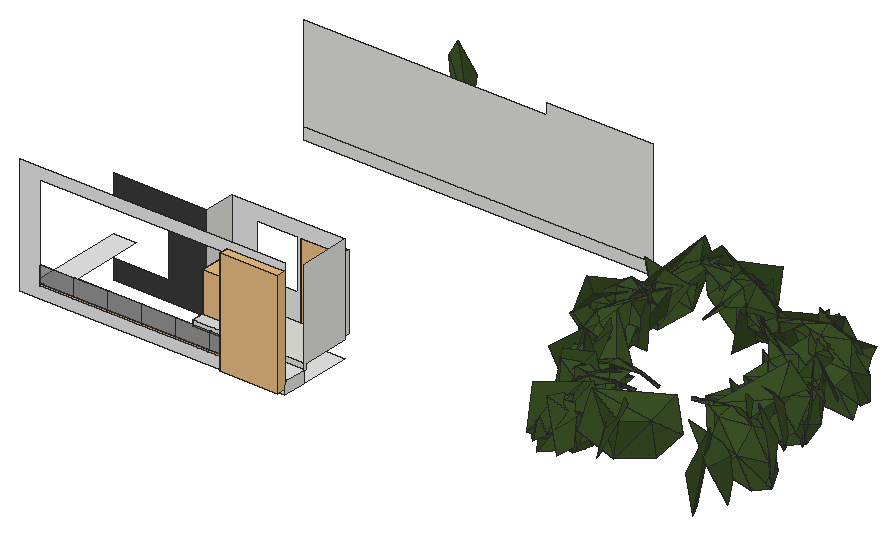
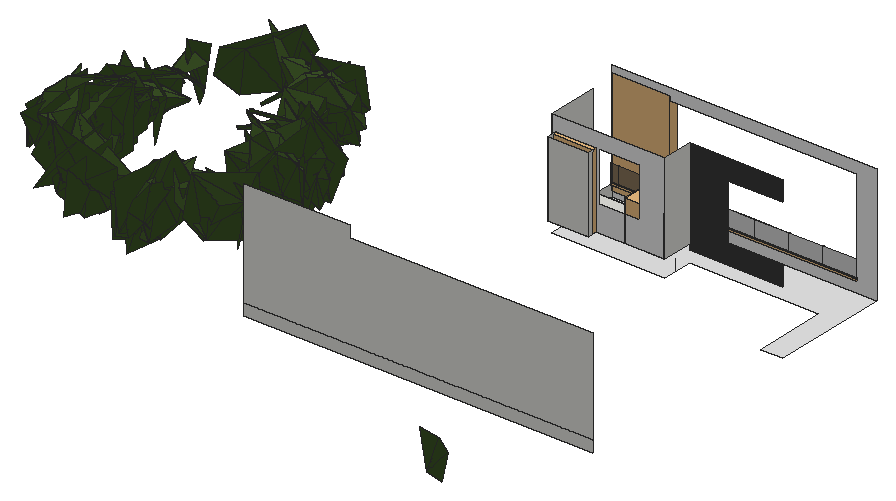
# SketchUp Ruby script. Lengths in inches.
U = 1.inch
M = Sketchup.active_model
def pt(a) = Geom::Point3d.new(a.map { |v| v * U })
def face(e, loops, mat)
  f = e.add_face(loops[0].map { |a| pt(a) })
  loops[1..].each { |l| e.add_face(l.map { |a| pt(a) }).erase! }
  f.material = f.back_material = mat if mat
  f
end
# faces: each face lists its corners as indices into pts; further lists are holes
def faces(e, pts, list, mat = nil) = list.each { |f| face(e, (f[0].is_a?(Array) ? f : [f]).map { |l| l.map { |i| pts[i] } }, mat) }
# xy, xz, yz: faces in a plane at the given z, y or x. An outline is a flat list of corners, or four numbers for a rectangle; further outlines are holes
def ring(l) = l.size == 4 ? [[l[0], l[1]], [l[2], l[1]], [l[2], l[3]], [l[0], l[3]]] : l.each_slice(2).to_a
def flat(e, list, mat, &to3) = list.each { |f| face(e, (f[0].is_a?(Array) ? f : [f]).map { |l| ring(l).map { |u, v| to3.(u, v) } }, mat) }
def xy(e, z, list, mat = nil) = flat(e, list, mat) { |x, y| [x, y, z] }
def xz(e, y, list, mat = nil) = flat(e, list, mat) { |x, z| [x, y, z] }
def yz(e, x, list, mat = nil) = flat(e, list, mat) { |y, z| [x, y, z] }
def lines(e, pts, list) = list.each { |a, b| e.add_line(pt(pts[a]), pt(pts[b])) }
# prism: a flat outline (further loops are holes) pulled along v
def prism(e, loops, v, mat = nil)
  f = face(e, loops, mat); d = Geom::Vector3d.new(v.map { |x| x * U })
  f.pushpull(f.normal.samedirection?(d) ? d.length : -d.length)
end
def box(e, o, s, mat = nil) = prism(e, [[o, [o[0] + s[0], o[1], o[2]], [o[0] + s[0], o[1] + s[1], o[2]], [o[0], o[1] + s[1], o[2]]]], [0, 0, s[2]], mat)
def at(x, y, z, deg = 0) = Geom::Transformation.translation(pt([x, y, z])) * Geom::Transformation.rotation(ORIGIN, Z_AXIS, deg.degrees)
def axes(o, x, y, z) = Geom::Transformation.new([*x, 0, *y, 0, *z, 0, *pt(o).to_a, 1])
def part(name) = M.definitions.add(name)
# library, detail: a bought-in or finely detailed component or shape, given as its bounding box
def library(name, o, s) = part(name).tap { |d| box(d.entities, o, s) }
def detail(e, o, s) = box(e.add_group.entities, o, s)
def put(e, d, t, mat = nil) = e.add_instance(d, t).tap { |i| i.material = mat if mat }
def group(e, t, mat = nil) = e.add_group.tap { |g| g.transformation = t; g.material = mat if mat }.entities
root = M.entities
M.materials.add("AM113_062_Tilia").color = [58, 81, 37]
M.materials.add("[Color M07]").color = [58, 58, 58]
M.materials.add("[Translucent_Glass_Blue]").color = [63, 63, 63]
M.materials["[Translucent_Glass_Blue]"].alpha = 0.35
M.materials.add("metal railing").color = [165, 165, 165]
M.materials.add("plastic2").color = [86, 86, 86]
M.materials.add("white_wall").color = [233, 233, 233]
c1 = library("Railing",[0,0,0],[72,2.52,4.03])
c2 = part("railing plastic")
box(c2.entities,[0,0.75,0],[72,0.26,0.68],"plastic2")
box(c2.entities,[0,0,0],[72,0.26,0.68],"plastic2")
c3 = part("Glass Railing pro")
put(c3.entities,c1,axes([0,0,0],[7.25965,0,0],[0,1,0],[0,0,1]))
put(c3.entities,c2,axes([0,0.75,3.47],[7.25965,0,0],[0,1,0],[0,0,1]))
c4 = part("sheet glass")
box(c4.entities,[0,0,0],[39.37,0.39,39.37],"[Translucent_Glass_Blue]")
c5 = part("glass stretch")
box(c5.entities,[0,0,0],[39.37,0.39,43.31],"[Translucent_Glass_Blue]")
c6 = part("glass frame")
put(c6.entities,c4,axes([0,0,0],[1.8288,0,0],[0,1.016,0],[0,0,1]))
put(c6.entities,c5,axes([505.4,0,0],[0.43929,0,0],[0,1.016,0],[0,0,0.90909]))
put(c6.entities,c4,axes([72.2,0,0],[1.8288,0,0],[0,1.016,0],[0,0,1]))
put(c6.entities,c4,axes([144.4,0,0],[1.8288,0,0],[0,1.016,0],[0,0,1]))
put(c6.entities,c4,axes([216.6,0,0],[1.8288,0,0],[0,1.016,0],[0,0,1]))
put(c6.entities,c4,axes([288.8,0,0],[1.8288,0,0],[0,1.016,0],[0,0,1]))
put(c6.entities,c4,axes([361,0,0],[1.8288,0,0],[0,1.016,0],[0,0,1]))
put(c6.entities,c4,axes([433.2,0,0],[1.8288,0,0],[0,1.016,0],[0,0,1]))
c7 = part("Glass Railing +")
put(c7.entities,c3,at(0,0,0),"metal railing")
put(c7.entities,c6,at(0,1.0625,1.53),"metal railing")
c8 = part("My+Glass_Railing")
put(c8.entities,c7,at(-0.34,0,0))
c9 = library("plant (1)",[-21.34,-27.21,-0.38],[41.91,41.15,38.97])
c10 = library("Shrub+_Grass",[-121.83,-22.34,0],[123.96,19.94,123.95])
c11 = library("PINTU+6+YA",[0,-0.6875,0],[35.83,8.07,80.71])
xy(root,273.04,[[371.87,28.625,371.87,278.26,418.81,278.26,418.81,121.6875,695.48,121.6875,695.48,187.1875,935.92,187.1875,935.92,28.625]],"white_wall")
xy(root,308.91,[[695.48,83.29,935.92,83.29,935.92,187.1875,927.68,187.1875,927.68,207.4375,841.77,207.4375,841.77,187.1875,695.48,187.1875]])
xz(root,28.625,[[371.87,273.04,935.92,273.04,935.92,297.35,413.32,297.35,413.32,500.91,935.92,500.91,935.92,525.1,371.87,525.1]],"white_wall")
xz(root,83.29,[[695.48,297.35,935.92,308.91]])
xz(root,121.6875,[[496.21,297.35,695.48,297.35,695.48,500.91,496.21,500.91,496.21,457.89,613.65,457.89,613.65,339.36,496.21,339.36]],"[Color M07]")
xz(root,187.1875,[[695.48,308.91,841.77,308.91,841.77,469.24,835.24,469.24,835.24,364.43,748.74,364.43,748.74,469.24,927.68,469.24,927.68,308.91,935.92,308.91,935.92,500.91,695.48,500.91]],"white_wall")
xz(root,207.4375,[[841.77,308.91,927.68,469.24]])
xz(root,725.65,[[418.81,273.04,1160.625,297.35],[418.81,297.35,418.81,500.91,935.92,500.91,935.92,525.1,1160.625,525.1,1160.625,297.35]])
yz(root,695.48,[[83.29,297.35,121.6875,308.91],[121.6875,308.91,187.1875,500.91]])
yz(root,841.77,[[187.1875,308.91,207.4375,469.24]])
yz(root,927.68,[[187.1875,308.91,207.4375,469.24]])
yz(root,935.92,[[28.625,273.04,76.875,297.35],[76.875,297.35,76.875,500.91,187.1875,500.91,187.1875,308.91,83.29,308.91,83.29,297.35]])
p = [[1726.04,425.28,347.14],[1633.73,427.27,429.39],[1677.65,428,251.14],[1612.37,455.72,310.63],[1284.72,331.65,346.32],[1334.89,406.05,429.43],
  [1303.44,377.73,253.56],[1361.71,418.12,309.96],[1703.03,155.11,256.72],[1686.97,186.29,255.56],[1681.79,228.74,364.75],[1365.41,276.39,256.16],
  [1387.28,221.24,314.07],[1379.55,269.8,365.5],[1360.82,315.08,327.84],[1397.36,380.08,315.61],[1345.32,356.24,258.76],[1690.04,216.5,392.49],
  [1699.77,139.08,344.57],[1721.375,172.58,346.28],[1726.25,219.67,257.36],[1704.02,272.17,325.3],[1717.7,253.93,333.4375],[1741.12,263.69,269.3],
  [1749.15,306.62,257.48],[1745.96,302.05,307.52],[1737.48,337.56,274.56],[1758.18,295.16,270.1],[1723.52,296.66,263.39],[1676.53,340.13,353.67],
  [597.55,943.93,270.1],[562.89,945.4375,263.39],[515.91,988.9,353.67],[1428.98,246.7,383.67],[1431.46,209.37,265.86],[1381.28,141.36,270.84],
  [1342.81,341.56,313.11],[1318.22,305.65,268.03],[1318.72,262.98,284.91],[1357.34,354.46,274.22],[1301.16,337.16,269.15],[1322.875,316.55,292.7],
  [1288.6,336.99,316.2],[1276.45,388.35,348.44],[1280.3,374.92,279.89],[1696.57,232,309],[1600.74,380.24,382.82],[1642.35,361.07,270.04],
  [1696.99,298.53,290.85],[1689.04,347.97,381.4],[1763.05,306.88,358.94],[528.41,996.75,381.4],[602.42,955.65,358.94],[1679.3,390.71,342.86],
  [1690.81,406.47,275.41],[1714.71,443.96,270.55],[1719.99,428.79,316.66],[1722.2,471.07,298.74],[1393.48,140.27,384.3125],[1301.2,301.36,352.37],
  [1350.83,325.49,273.55],[1396.78,333.4,351.65],[1470.81,570.52,383.75],[1429.89,600.59,274.58],[1442.08,684.31,273.91],[1451.84,681.07,387.71],
  [1407.09,344.35,313.43],[1716.59,344.22,341.74],[1679.02,375.96,340.52],[1450.08,141.61,377.59],[1398.19,150.79,345.67],[1433.36,171.22,274.86],
  [1493.32,149.93,318.77],[1356.96,199,367.41],[1352.15,178.13,289],[1707.07,471.59,421.7],[1747.09,414.05,356.48],[1719.76,427.52,275.13],
  [1687.28,476.17,400.61],[1689.53,443.21,285.93],[1646.43,385.33,325.7],[1338.36,322.47,413.4],[1265.81,318.08,356.36],[1284.91,340.12,275.76],
  [1350.19,338.7,392.76],[1313.27,358.45,285.1],[1579.47,670.33,379.39],[1600.1875,656.35,276.45],[1549.98,598.59,293.16],[1631.46,604.85,285.62],
  [1559.9,610.85,276.43],[1568.6875,638.62,349.05],[1514.9,622.74,311.54],[1640.95,624.18,294.44],[1568.94,637.52,277.53],[1570.34,627.16,358.07],
  [1522.17,639.52,309.81],[1676.7,375.7,357.375],[1660.27,387.38,278.41],[1646.98,467.65,293.93],[1308.26,276.26,291.07],[1341.96,277.58,278.61],
  [1402.26,280.86,372.95],[1507.2,646.41,353.86],[1487.34,665.98,278.91],[1412.2,633.41,288.58],[1416.23,156.82,278.97],[1477.17,126.84,318.15],
  [1448.93,154.68,381.79],[1399.95,178.18,359.37],[1383.45,251.52,359.07],[1350.8125,202.68,304.82],[1335.69,376,279.71],[1375.93,318.09,305.31],
  [1338.23,326.37,368.4375],[1303.43,369.125,354.66],[1300.6875,433.48,401.69],[1277.03,424.43,315.95],[1286.06,420.29,333.45],[1626.25,386.16,394.92],
  [1647.42,376.84,306.64],[1663.15,455.26,281.29],[1683.37,423.34,354.01],[1704.53,473.5,375.93],[1695.01,516.46,317.22],[1745.05,453.86,358.01],
  [1701.11,493.34,281.66],[1670.37,523.71,364.83],[1631.55,298.57,384.19],[1653.92,280.43,309.82],[1679.53,355.7,282.71],[1688.625,325.45,360.85],
  [1707.99,377.21,384.49],[1712.01,414,318.11],[1337.61,244.41,315.62],[1323.84,286.14,325.15],[1626.29,642.77,358.61],[1659.9,612.78,420.2],
  [1693.04,625.34,350.76],[1265.67,396.73,364.82],[1278.3,410.02,286.46],[1354.74,383.57,290.86],[1333.87,265.93,379.5],[1358.04,229.11,287.8],
  [1425.96,237.375,335.07],[1359.11,624.36,350.54],[1402.9,652.98,396.73],[1445.66,669.03,350.16],[1365.61,466.4,442.68],[1362.47,458.08,317.86],
  [1294.15,500.29,289.38],[1264.375,490.23,394.64],[1507.4375,587.51,346.6],[1502.76,645.22,290.875],[1420.9,654.25,289.6],[1459.36,644.27,360.57],
  [1362.07,652.33,348.3125],[1410.72,642.07,398.875],[1696.26,323.0625,400.95],[1338.21,317.02,356.21],[1300.85,352.66,324.09],[1394.3,331.24,326.08],
  [1393.36,282.625,404.49],[1311.26,298.71,376.5625],[1586.78,334.52,365.78],[1629.1,286.26,323.04],[1689.5,336.53,291.24],[1661.83,334.64,371.14],
  [1694.84,379.4,387.43],[1730.85,393.36,322.73],[1371.56,309.83,382.64],[1325.54,314.99,364.36],[1580.39,552.54,388.88],[1603.34,547.19,406.0625],
  [1644.08,568.63,293.45],[1669.96,648.76,303.9375],[1699.92,431.54,324.46],[1713.14,479,364.5],[1673.99,524.74,338.95],[1624.26,618,378.92],
  [1651.8125,554.25,416.06],[1692.11,604.43,373.72],[1683.72,491.14,457.67],[1680.11,483.375,330.84],[1751.99,519.32,296.72],[1756.04,562.66,396.58],
  [1309.53,552.59,298.59],[1291.13,509.08,332.11],[1288.58,562.92,374.61],[1330.15,621.02,311.48],[1419.92,120.6,400.81],[1446.1875,114.86,298.66],
  [1498.94,163.25,337.35],[1720.91,467.99,371.51],[1702.98,509.82,395.58],[1490.33,652.09,345.54],[1497.02,634.4,306.22],[1464.87,688.15,301.48],
  [1424.85,702.36,319.19],[1285.33,566.55,303.35],[1276.0625,519.53,332.79],[1300.65,561.86,382.35],[1313.6875,633.61,323.1],[1741.4375,594.81,398.83],
  [1706.35,576.48,303.81],[1645.15,571.83,365.09],[1611.77,658.35,389.6],[1379.81,116.64,320.9],[1401.83,140.77,304.42],[1459.89,177.53,388.73],
  [1367.29,186.79,354.34],[1364.61,146.5,304.625],[1395.01,114.1,310.03],[1363.39,208.4,317.74],[1382.74,285.22,356.98],[1309.34,467.82,306.13],
  [1276.86,405.77,333.8],[1283.23,437.39,402.59],[1306.39,487.35,388.46],[1372.47,511.04,418.71],[1338.91,537.02,345.08],[1470.54,590.86,345],
  [1261.59,578.08,409.14],[1273.07,600.84,306.4],[1320.55,539.67,313.2],[1708.34,308.03,363.52],[1244.3,462.61,403.31],[1268.21,434.53,308.36],
  [1307.24,388.53,368.88],[1495.8,212.39,413.37],[1506.77,157.3,308.68],[1549.82,89.46,342.82],[1654.68,265.15,341.8125],[1325.18,452.46,309.81],
  [1299.36,392.34,345.54],[1272.41,434.84,393.14],[1284.64,486.03,363.83],[1319.62,531.72,401.77],[1320.61,532.91,319.94],[1513.89,578.59,351.68],
  [1425.9,110.98,332.54],[1390.64,132.27,354.46],[1720.6875,346.23,414.84],[1736.3,358.63,310.08],[1699.57,424.43,334.06],[1543.31,144.72,313.49],
  [1593.27,196.75,311.05],[1596.26,179.51,389.64],[1623.7,228.21,351.67],[1296.54,619.63,388.18],[1519.18,614.77,380.97],[1336.27,643.62,448.04],
  [1326.33,681.99,382.49],[1720.23,460.48,440.05],[1761.23,468.59,364.04],[1715.39,523.85,311.98],[1732.69,526.5,396.56],[1676.14,585.94,327.23],
  [1699.75,572.92,401.12],[1440.99,707.46,325.22],[1430.38,675.5625,312.32],[1413.22,616.86,405.83],[1365.09,307.53,369.4],[1408.37,343.0625,351.14],
  [1377.43,555.7,404.96],[1508.41,129.44,444.4375],[1509.76,89.54,379.18],[1562.47,132.39,396.57],[1398.6,211.61,379.8125],[1259.97,484.75,314.8],
  [1253.93,454.58,336.5],[1264.62,491.67,363.4],[1312.74,520.12,385.16],[1288.51,517.74,321.61],[1758.59,504.51,398.18],[1769.66,519.49,330.3125],
  [1754.78,559.875,315.06],[1757.74,558.1,365.41],[1730.71,582.48,332.27],[1363.37,266.92,373.65],[1406.58,244.64,383.27],[1446.73,257.97,404.6],
  [1306.13,346.31,384.94],[1701.86,434,387.08],[1720.09,533.73,373.32],[1413.11,231.55,346.4],[1502.54,123.21,378.12],[1725.57,437.68,378.09],
  [1513.07,137.98,381.62],[1445.11,689.04,358.91],[1401.12,690.78,350.03],[1457.39,171.02,421.14],[1381.79,130.13,409.52],[1341.89,525.52,360.42],
  [1737.7,423.93,378.02],[1321.58,611.83,405.38],[1391.59,624.58,436.63],[1347.98,675.87,402.84],[1418.25,624.22,437.4375],[1461.71,695.875,410.22],
  [1627.13,239.63,376.58],[1632.3,421.58,383.2],[1393.87,292.43,372.79],[1662.17,619.06,377.62],[1749.29,473.4,378.51],[1304.01,508.23,400.51],
  [1714.01,583.25,401.89],[1665.8,592.7,405.11],[1440.14,141.29,391.25],[1487.92,152.86,388.86],[1336.51,497.51,366.84],[1658.52,279.97,374.03],
  [1327.66,412.53,385.09],[1259.99,381.61,389.49],[1618.77,400.43,383.12],[1434.15,326.86,363.21],[1283.15,399.16,411.18],[1267.64,444.78,404.89],
  [1452.5,233.51,386.62],[1707.97,538.82,389.81],[1654.36,337.52,341.62],[1668.16,329.16,373.27],[1577.76,137.21,432.45],[1648.77,425.17,414.11],
  [1485.83,335.58,344.57],[1444.57,336.81,358.36],[1448.86,335.05,365.24],[1487.38,336.27,349.57],[1469.2,589.69,382.72],[1273.59,372.875,399.88],
  [1451.15,642.43,402.21],[1421.1,229.16,382.625],[1451.87,329.92,363.01],[1486.27,333.11,346.5],[1376.54,582.8,437.36],[1349.65,644.34,414.09],
  [1325.07,394.86,414.3],[1377.86,625.31,416.8],[1413.73,658.16,407.28],[1348.15,626.4,418.59],[1406.25,326.25,378.875],[1602.91,235.8,416.02],
  [1353.33,386.83,428.46],[1391.97,619.13,459.49],[1414.78,172.88,397.31],[1422.6,281.88,356.1],[1409.27,298.91,381.73],[1359.29,300.94,424.68],
  [1395.04,323.5,428.45],[1716.01,499.5,437.51],[1642.04,452.92,432.33],[1512.61,188.14,407.47],[1360.07,479.74,400.53],[1292.86,472.96,422.3125],
  [1482.08,275.44,363.5],[1453.06,248.12,382.99],[1458.49,249.24,388.64],[1483.61,276.6875,368.32],[1666.68,303.91,387.53],[1368.27,354.18,391.28],
  [1345.47,349.93,413.5625],[1463.61,247.56,384.74],[1484.3,273.79,364.68],[1667.59,512.39,451.78],[1726.09,549.37,426.71],[1675.63,451.03,398.31],
  [1485.92,161.66,434.49],[1354.79,442.08,441.4],[1471.51,192.83,369.74],[1455,195.08,400.94],[1583.29,300.37,371.29],[1625.1,295.55,380],
  [1622.08,300.42,385.33],[1582.32,301.88,376.23],[1619.62,304.68,380.49],[1583.47,303.28,371.48],[1679.11,464.81,420],[1664.76,485,399.64],
  [1678.55,520.23,443.11],[1447.6875,554.38,396.46],[1435.27,518.03,380.29],[1435.12,519.78,375.32],[1450.78,557.86,389.6],[1441.82,553.37,394.3],
  [1432.68,520.2,377.29],[1632.49,580.51,441.6875],[1694.29,422.65,432.41],[1699.02,484.55,416.1],[1434.84,213.57,405.61],[1454.42,597.22,410.8],
  [1328.98,369.56,425.16],[1349.05,472.3,433.54],[1669.28,439.77,427.96],[1406.94,597.62,388.7],[1427.77,603.89,414.16],[1312.9,378.94,445.43],
  [1279.07,402.82,457],[1697.34,501.72,446.64],[1663.3,547.42,412.1875],[1681.57,549.15,441.77],[1323.49,419,409.6],[1315.89,435.93,438.2],
  [1366.27,395.25,439.63],[1628.51,449.59,439.08],[1357.21,399.72,435.96],[1628.0625,459.46,444.23],[1329.88,457.65,449.04],[1360.86,396.82,442.625],
  [1693.64,527.51,457.45],[1629.21,453.64,446.49],[1369.23,442.97,444.42],[1393.26,419.47,446.92],[1369.2,432.61,446.56],[1593.27,471.3,452.24],
  [1393.6,418.22,452.02],[1394.69,417,447.26],[1369.26,437.87,450.52],[1402.08,415.74,445.45],[1402.07,417.03,440.34],[1400.4375,414.71,440.875],
  [1651.95,504.99,458.05],[1594.125,471.76,457.55],[1594.78,473.73,452.98],[1661.14,499.64,457.15],[1656.51,502.82,462.67],[1620.67,484.27,460.01],
  [1621.9,483.05,455.03],[1620.66,485.68,455.04],[695.48,160.1875,297.35],[695.48,160.1875,273.04]]
faces(root,p,[[0,1,2],[1,3,2],[4,5,6],[5,7,6],[8,9,10],[11,12,13],[13,14,11],[15,16,11],
  [11,14,15],[17,18,8],[10,17,8],[19,20,21],[22,23,24],[24,25,22],[24,26,25],[27,28,29],
  [30,31,32],[33,34,35],[36,37,38],[36,39,37],[40,41,42],[40,42,43],[43,44,40],[22,45,23],
  [46,47,48],[29,49,27],[49,50,27],[32,51,30],[51,52,30],[53,54,55],[55,56,53],[55,57,56],
  [58,33,35],[59,60,61],[62,63,64],[65,62,64],[66,39,36],[25,26,67],[26,68,67],[69,70,71],
  [71,72,69],[71,70,73],[73,74,71],[75,76,77],[78,75,77],[77,79,78],[53,80,54],[81,82,83],
  [84,81,83],[83,85,84],[86,87,88],[89,90,91],[90,92,91],[93,94,95],[94,96,95],[97,98,99],
  [100,101,102],[103,104,105],[106,107,108],[108,109,106],[110,111,106],[106,109,110],[112,113,114],[114,115,112],
  [112,115,116],[116,117,112],[43,118,44],[119,120,121],[121,122,119],[123,122,121],[121,124,123],[125,126,127],
  [128,129,130],[130,131,128],[132,131,130],[130,133,132],[38,134,135],[38,135,36],[91,136,89],[89,136,137],
  [137,138,89],[139,140,141],[142,143,144],[105,145,146],[146,147,105],[105,147,103],[148,149,150],[151,148,150],
  [152,153,154],[154,155,152],[154,156,157],[157,155,154],[158,46,48],[159,160,141],[141,161,159],[141,160,139],
  [102,162,100],[162,163,100],[164,165,166],[166,167,164],[168,167,166],[166,169,168],[41,170,171],[42,41,171],
  [86,88,172],[173,174,175],[99,176,97],[177,176,99],[99,178,177],[93,179,180],[180,181,93],[95,179,93],
  [182,183,184],[185,182,184],[186,187,188],[189,186,188],[190,191,192],[56,57,193],[57,194,193],[195,196,197],
  [195,197,198],[199,200,201],[202,199,201],[203,204,205],[206,173,175],[207,208,209],[210,211,212],[210,213,211],
  [113,214,114],[215,216,217],[217,218,215],[215,218,219],[219,220,215],[221,196,195],[222,223,224],[22,25,225],
  [225,25,67],[226,227,228],[229,230,231],[232,45,22],[233,234,235],[235,236,233],[233,236,237],[237,238,233],
  [95,96,239],[212,240,241],[212,241,210],[242,243,244],[245,246,247],[246,248,247],[188,249,189],[91,92,250],
  [189,249,251],[251,252,189],[253,254,255],[255,256,253],[255,257,258],[258,256,255],[259,260,261],[36,135,262],
  [263,36,262],[36,263,66],[222,224,264],[265,266,245],[245,267,265],[247,267,245],[12,268,13],[269,270,271],
  [272,273,269],[269,271,272],[274,275,276],[276,277,274],[276,278,277],[135,134,279],[134,280,279],[13,281,15],
  [15,14,13],[282,42,171],[43,42,282],[53,56,283],[283,56,193],[124,284,123],[285,213,210],[107,286,108],
  [133,287,132],[72,288,69],[198,289,195],[198,290,289],[209,291,207],[291,292,207],[272,293,273],[169,294,168],
  [201,295,202],[202,295,296],[296,297,202],[139,160,159],[97,176,177],[262,135,279],[261,298,259],[298,299,259],
  [19,21,300],[301,80,53],[161,302,159],[257,303,258],[274,304,275],[188,187,305],[277,278,306],[278,307,306],
  [241,240,308],[240,309,308],[201,200,310],[22,311,232],[311,22,225],[312,118,43],[216,313,217],[242,244,314],
  [142,144,315],[270,316,317],[271,270,317],[190,192,318],[178,319,177],[67,68,320],[320,321,67],[225,67,321],
  [322,229,231],[53,323,301],[323,53,283],[324,325,326],[326,327,324],[195,328,221],[234,329,235],[328,195,330],
  [195,289,330],[73,70,69],[210,331,285],[332,333,327],[157,334,152],[152,155,157],[156,335,157],[336,43,282],
  [43,336,312],[91,250,137],[137,136,91],[327,326,332],[290,337,338],[289,290,338],[103,147,146],[145,339,146],
  [262,340,263],[325,263,340],[247,248,341],[59,61,342],[95,239,180],[146,343,103],[119,122,123],[210,241,344],
  [331,210,344],[344,241,308],[116,115,114],[279,280,345],[345,346,279],[159,302,347],[159,347,139],[114,214,348],
  [177,349,97],[125,127,350],[180,179,95],[340,326,325],[330,289,338],[108,351,110],[110,109,108],[352,293,272],
  [128,131,132],[340,346,332],[332,326,340],[353,271,317],[272,271,353],[354,355,356],[356,357,354],[225,358,311],
  [225,321,358],[237,236,235],[171,170,359],[282,171,360],[359,360,171],[177,319,349],[361,362,357],[203,205,363],
  [274,277,364],[364,277,306],[13,268,281],[168,365,164],[164,167,168],[201,310,296],[69,366,73],[357,356,361],
  [114,348,116],[226,228,367],[262,279,346],[262,346,340],[308,309,368],[368,369,308],[370,371,372],[372,373,370],
  [374,375,373],[283,193,376],[377,376,193],[193,194,377],[358,321,374],[123,284,378],[371,311,358],[188,305,251],
  [251,249,188],[379,380,381],[381,382,379],[123,378,119],[373,372,374],[383,384,380],[69,288,366],[258,303,385],
  [168,294,365],[108,286,351],[132,287,386],[387,304,274],[358,372,371],[380,379,383],[374,372,358],[296,295,201],
  [344,388,331],[355,331,388],[382,328,389],[330,389,328],[388,356,355],[132,386,128],[388,369,361],[361,356,388],
  [282,360,390],[282,390,336],[391,272,353],[272,391,352],[283,392,323],[283,376,392],[219,218,217],[338,337,393],
  [393,394,338],[217,313,395],[247,341,265],[265,267,247],[389,379,382],[344,308,369],[235,329,396],[235,396,237],
  [389,394,383],[383,379,389],[253,256,258],[146,339,343],[344,369,388],[274,397,387],[397,274,364],[157,335,334],
  [258,385,253],[306,307,398],[398,399,306],[364,306,399],[330,394,389],[330,338,394],[217,395,219],[317,316,400],
  [400,401,317],[353,317,401],[390,360,402],[403,323,392],[404,336,390],[392,376,405],[353,401,406],[353,406,391],
  [402,407,390],[390,407,404],[364,408,397],[364,399,408],[405,409,392],[392,409,403],[410,391,406],[411,404,407],
  [406,401,412],[413,403,409],[414,407,402],[402,415,414],[416,417,418],[418,410,416],[412,419,417],[408,399,420],
  [407,414,411],[421,409,405],[405,422,421],[406,416,410],[417,416,412],[409,421,413],[412,416,406],[423,397,408],
  [424,425,426],[426,423,424],[420,427,425],[408,424,423],[420,424,408],[425,424,420]],"AM113_062_Tilia")
lines(root,p,[[428,429]])
put(root,c8,at(413.5625,28.625,297.35))
put(root,c9,axes([740.02,160.01,309.75],[2.0178,0,0],[0,1.9494,0],[0,0,2.1888]))
put(root,c10,axes([933.79,31.03,284.22],[1,0,0],[0,1,0],[0,0,1.815]))
put(root,c11,axes([841.77,187.1875,308.91],[2.3979,0,0],[0,1,0],[0,0,1.9865]))
